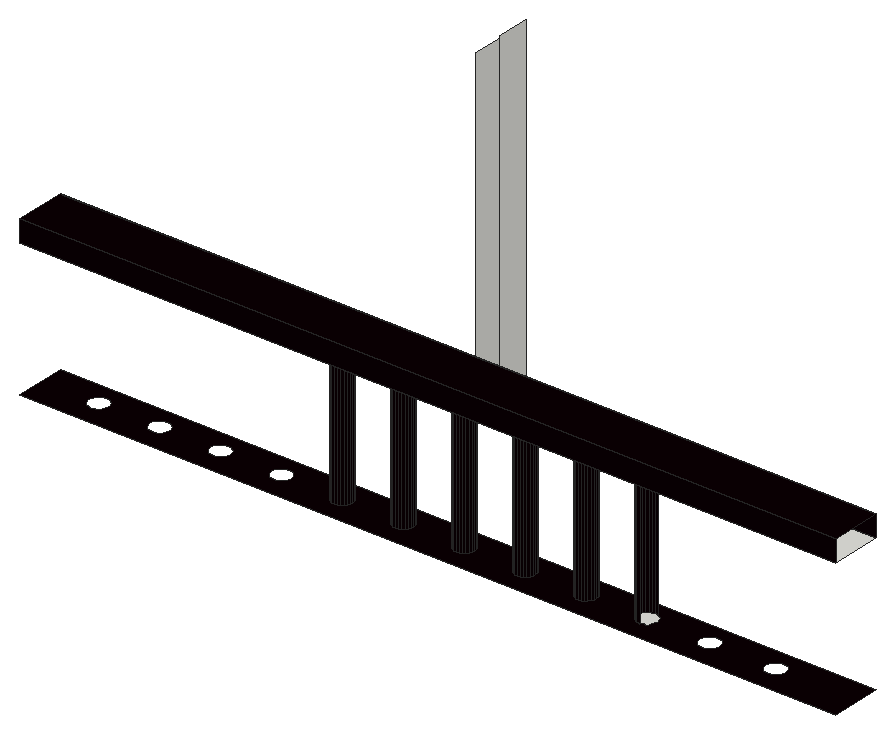
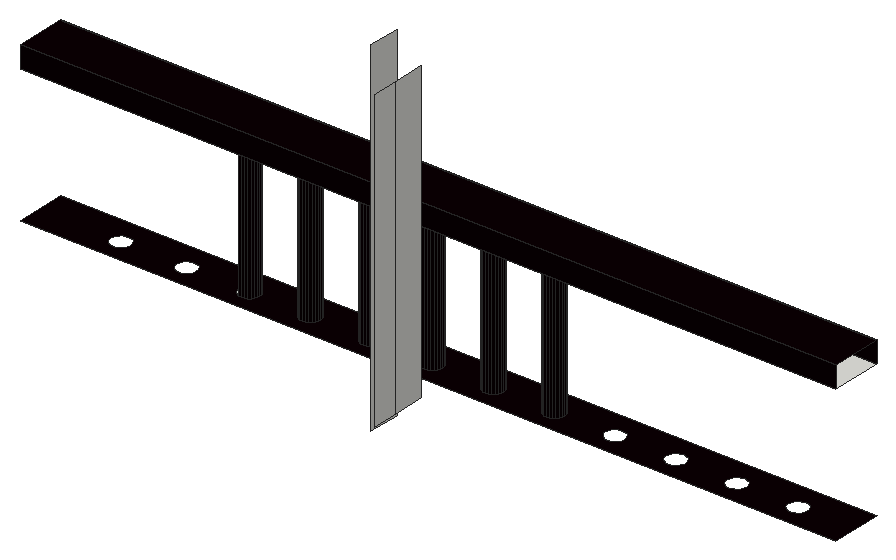
# SketchUp Ruby script. Lengths in inches.
U = 1.inch
M = Sketchup.active_model
def pt(a) = Geom::Point3d.new(a.map { |v| v * U })
def face(e, loops, mat)
  f = e.add_face(loops[0].map { |a| pt(a) })
  loops[1..].each { |l| e.add_face(l.map { |a| pt(a) }).erase! }
  f.material = f.back_material = mat if mat
  f
end
# faces: each face lists its corners as indices into pts; further lists are holes
def faces(e, pts, list, mat = nil) = list.each { |f| face(e, (f[0].is_a?(Array) ? f : [f]).map { |l| l.map { |i| pts[i] } }, mat) }
# xy, xz, yz: faces in a plane at the given z, y or x. An outline is a flat list of corners, or four numbers for a rectangle; further outlines are holes
def ring(l) = l.size == 4 ? [[l[0], l[1]], [l[2], l[1]], [l[2], l[3]], [l[0], l[3]]] : l.each_slice(2).to_a
def flat(e, list, mat, &to3) = list.each { |f| face(e, (f[0].is_a?(Array) ? f : [f]).map { |l| ring(l).map { |u, v| to3.(u, v) } }, mat) }
def xy(e, z, list, mat = nil) = flat(e, list, mat) { |x, y| [x, y, z] }
def xz(e, y, list, mat = nil) = flat(e, list, mat) { |x, z| [x, y, z] }
def yz(e, x, list, mat = nil) = flat(e, list, mat) { |y, z| [x, y, z] }
def lines(e, pts, list) = list.each { |a, b| e.add_line(pt(pts[a]), pt(pts[b])) }
# prism: a flat outline (further loops are holes) pulled along v
def prism(e, loops, v, mat = nil)
  f = face(e, loops, mat); d = Geom::Vector3d.new(v.map { |x| x * U })
  f.pushpull(f.normal.samedirection?(d) ? d.length : -d.length)
end
def box(e, o, s, mat = nil) = prism(e, [[o, [o[0] + s[0], o[1], o[2]], [o[0] + s[0], o[1] + s[1], o[2]], [o[0], o[1] + s[1], o[2]]]], [0, 0, s[2]], mat)
def at(x, y, z, deg = 0) = Geom::Transformation.translation(pt([x, y, z])) * Geom::Transformation.rotation(ORIGIN, Z_AXIS, deg.degrees)
def axes(o, x, y, z) = Geom::Transformation.new([*x, 0, *y, 0, *z, 0, *pt(o).to_a, 1])
def part(name) = M.definitions.add(name)
# library, detail: a bought-in or finely detailed component or shape, given as its bounding box
def library(name, o, s) = part(name).tap { |d| box(d.entities, o, s) }
def detail(e, o, s) = box(e.add_group.entities, o, s)
def put(e, d, t, mat = nil) = e.add_instance(d, t).tap { |i| i.material = mat if mat }
def group(e, t, mat = nil) = e.add_group.tap { |g| g.transformation = t; g.material = mat if mat }.entities
root = M.entities
M.materials.add("[Metal Seamed]").color = [11, 0, 4]
xy(root,300,[[437.97,74.99,437.36,75.05,436.8,75.25,436.3,75.6,435.91,76.06,435.66,76.61,435.55,77.2,435.6,77.8,435.81,78.37,436.16,78.86,436.62,79.25,437.16,79.51,437.76,79.61,438.36,79.5625,438.93,79.36,439.42,79.01,439.8125,78.55,440.07,78,440.17,77.41,440.12,76.81,439.91,76.24,439.57,75.74,439.11,75.36,438.56,75.1],[451.9,74.99,451.3,75.05,450.73,75.25,450.24,75.6,449.85,76.06,449.6,76.61,449.49,77.2,449.54,77.8,449.75,78.37,450.09,78.86,450.56,79.25,451.1,79.51,451.7,79.61,452.3,79.5625,452.87,79.36,453.36,79.01,453.75,78.55,454,78,454.11,77.41,454.06,76.81,453.85,76.24,453.51,75.74,453.04,75.36,452.5,75.1],[465.84,74.99,465.24,75.05,464.67,75.25,464.18,75.6,463.79,76.06,463.53,76.61,463.43,77.2,463.48,77.8,463.69,78.37,464.03,78.86,464.49,79.25,465.04,79.51,465.63,79.61,466.24,79.5625,466.8,79.36,467.3,79.01,467.6875,78.55,467.94,78,468.05,77.41,468,76.81,467.79,76.24,467.44,75.74,466.98,75.36,466.44,75.1],[479.78,74.99,479.18,75.05,478.61,75.25,478.11,75.6,477.73,76.06,477.47,76.61,477.36,77.2,477.42,77.8,477.62,78.37,477.97,78.86,478.43,79.25,478.98,79.51,479.57,79.61,480.17,79.5625,480.74,79.36,481.24,79.01,481.625,78.55,481.88,78,481.99,77.41,481.93,76.81,481.73,76.24,481.38,75.74,480.92,75.36,480.37,75.1],[493.72,74.99,493.11,75.05,492.55,75.25,492.05,75.6,491.66,76.06,491.41,76.61,491.3,77.2,491.35,77.8,491.56,78.37,491.91,78.86,492.37,79.25,492.91,79.51,493.51,79.61,494.11,79.5625,494.68,79.36,495.17,79.01,495.5625,78.55,495.82,78,495.92,77.41,495.87,76.81,495.66,76.24,495.32,75.74,494.86,75.36,494.31,75.1],
  [507.65,74.99,507.05,75.05,506.48,75.25,505.99,75.6,505.6,76.06,505.35,76.61,505.24,77.2,505.29,77.8,505.5,78.37,505.84,78.86,506.31,79.25,506.85,79.51,507.45,79.61,508.05,79.5625,508.62,79.36,509.11,79.01,509.5,78.55,509.75,78,509.86,77.41,509.81,76.81,509.6,76.24,509.26,75.74,508.79,75.36,508.25,75.1]])
xy(root,300,[[[369.3125,70.97,555.7,82.57],[382.22,74.99,381.61,75.05,381.05,75.25,380.55,75.6,380.16,76.06,379.91,76.61,379.8,77.2,379.85,77.8,380.06,78.37,380.41,78.86,380.87,79.25,381.41,79.51,382.01,79.61,382.61,79.5625,383.18,79.36,383.67,79.01,384.0625,78.55,384.32,78,384.42,77.41,384.37,76.81,384.16,76.24,383.82,75.74,383.36,75.36,382.81,75.1],[396.15,74.99,395.55,75.05,394.98,75.25,394.49,75.6,394.1,76.06,393.85,76.61,393.74,77.2,393.79,77.8,394,78.37,394.34,78.86,394.81,79.25,395.35,79.51,395.95,79.61,396.55,79.5625,397.12,79.36,397.61,79.01,398,78.55,398.25,78,398.36,77.41,398.31,76.81,398.1,76.24,397.76,75.74,397.29,75.36,396.75,75.1],[410.09,74.99,409.49,75.05,408.92,75.25,408.43,75.6,408.04,76.06,407.78,76.61,407.68,77.2,407.73,77.8,407.94,78.37,408.28,78.86,408.74,79.25,409.29,79.51,409.88,79.61,410.49,79.5625,411.05,79.36,411.55,79.01,411.9375,78.55,412.19,78,412.3,77.41,412.25,76.81,412.04,76.24,411.69,75.74,411.23,75.36,410.69,75.1],[424.03,74.99,423.43,75.05,422.86,75.25,422.36,75.6,421.98,76.06,421.72,76.61,421.61,77.2,421.67,77.8,421.87,78.37,422.22,78.86,422.68,79.25,423.23,79.51,423.82,79.61,424.42,79.5625,424.99,79.36,425.49,79.01,425.875,78.55,426.13,78,426.24,77.41,426.18,76.81,425.98,76.24,425.63,75.74,425.17,75.36,424.62,75.1],[437.97,74.99,437.36,75.05,436.8,75.25,436.3,75.6,435.91,76.06,435.66,76.61,435.55,77.2,435.6,77.8,435.81,78.37,436.16,78.86,436.62,79.25,437.16,79.51,437.76,79.61,438.36,79.5625,438.93,79.36,439.42,79.01,439.8125,78.55,440.07,78,440.17,77.41,440.12,76.81,439.91,76.24,439.57,75.74,439.11,75.36,438.56,75.1],[451.9,74.99,451.3,75.05,450.73,75.25,450.24,75.6,449.85,76.06,449.6,76.61,449.49,77.2,449.54,77.8,449.75,78.37,450.09,78.86,450.56,79.25,451.1,79.51,451.7,79.61,452.3,79.5625,452.87,79.36,453.36,79.01,453.75,78.55,454,78,454.11,77.41,454.06,76.81,453.85,76.24,453.51,75.74,453.04,75.36,452.5,75.1],[465.84,74.99,465.24,75.05,464.67,75.25,464.18,75.6,463.79,76.06,463.53,76.61,463.43,77.2,463.48,77.8,463.69,78.37,464.03,78.86,464.49,79.25,465.04,79.51,465.63,79.61,466.24,79.5625,466.8,79.36,467.3,79.01,467.6875,78.55,467.94,78,468.05,77.41,468,76.81,467.79,76.24,467.44,75.74,466.98,75.36,466.44,75.1],[479.78,74.99,479.18,75.05,478.61,75.25,478.11,75.6,477.73,76.06,477.47,76.61,477.36,77.2,477.42,77.8,477.62,78.37,477.97,78.86,478.43,79.25,478.98,79.51,479.57,79.61,480.17,79.5625,480.74,79.36,481.24,79.01,481.625,78.55,481.88,78,481.99,77.41,481.93,76.81,481.73,76.24,481.38,75.74,480.92,75.36,480.37,75.1],[493.72,74.99,493.11,75.05,492.55,75.25,492.05,75.6,491.66,76.06,491.41,76.61,491.3,77.2,491.35,77.8,491.56,78.37,491.91,78.86,492.37,79.25,492.91,79.51,493.51,79.61,494.11,79.5625,494.68,79.36,495.17,79.01,495.5625,78.55,495.82,78,495.92,77.41,495.87,76.81,495.66,76.24,495.32,75.74,494.86,75.36,494.31,75.1],[507.65,74.99,507.05,75.05,506.48,75.25,505.99,75.6,505.6,76.06,505.35,76.61,505.24,77.2,505.29,77.8,505.5,78.37,505.84,78.86,506.31,79.25,506.85,79.51,507.45,79.61,508.05,79.5625,508.62,79.36,509.11,79.01,509.5,78.55,509.75,78,509.86,77.41,509.81,76.81,509.6,76.24,509.26,75.74,508.79,75.36,508.25,75.1],[521.97,74.99,521.36,75.05,520.8,75.25,520.3,75.6,519.91,76.06,519.66,76.61,519.55,77.2,519.6,77.8,519.81,78.37,520.16,78.86,520.62,79.25,521.16,79.51,521.76,79.61,522.36,79.5625,522.93,79.36,523.42,79.01,523.8125,78.55,524.07,78,524.17,77.41,524.12,76.81,523.91,76.24,523.57,75.74,523.11,75.36,522.56,75.1],[537.09,74.99,536.49,75.05,535.92,75.25,535.43,75.6,535.04,76.06,534.78,76.61,534.68,77.2,534.73,77.8,534.94,78.37,535.28,78.86,535.74,79.25,536.29,79.51,536.88,79.61,537.49,79.5625,538.05,79.36,538.55,79.01,538.9375,78.55,539.19,78,539.3,77.41,539.25,76.81,539.04,76.24,538.69,75.74,538.23,75.36,537.69,75.1]]],"[Metal Seamed]")
xy(root,331.08,[[[369.3125,70.97,555.7,82.57],[382.22,74.99,382.81,75.1,383.36,75.36,383.82,75.74,384.16,76.24,384.37,76.81,384.42,77.41,384.32,78,384.0625,78.55,383.67,79.01,383.18,79.36,382.61,79.5625,382.01,79.61,381.41,79.51,380.87,79.25,380.41,78.86,380.06,78.37,379.85,77.8,379.8,77.2,379.91,76.61,380.16,76.06,380.55,75.6,381.05,75.25,381.61,75.05],[424.03,74.99,424.62,75.1,425.17,75.36,425.63,75.74,425.98,76.24,426.18,76.81,426.24,77.41,426.13,78,425.875,78.55,425.49,79.01,424.99,79.36,424.42,79.5625,423.82,79.61,423.23,79.51,422.68,79.25,422.22,78.86,421.87,78.37,421.67,77.8,421.61,77.2,421.72,76.61,421.98,76.06,422.36,75.6,422.86,75.25,423.43,75.05]]])
xy(root,331.3125,[[451.9,74.99,452.5,75.1,453.04,75.36,453.51,75.74,453.85,76.24,454.06,76.81,454.11,77.41,454,78,453.75,78.55,453.36,79.01,452.87,79.36,452.3,79.5625,451.7,79.61,451.1,79.51,450.56,79.25,450.09,78.86,449.75,78.37,449.54,77.8,449.49,77.2,449.6,76.61,449.85,76.06,450.24,75.6,450.73,75.25,451.3,75.05]])
xy(root,331.6875,[[465.84,74.99,466.44,75.1,466.98,75.36,467.44,75.74,467.79,76.24,468,76.81,468.05,77.41,467.94,78,467.6875,78.55,467.3,79.01,466.8,79.36,466.24,79.5625,465.63,79.61,465.04,79.51,464.49,79.25,464.03,78.86,463.69,78.37,463.48,77.8,463.43,77.2,463.53,76.61,463.79,76.06,464.18,75.6,464.67,75.25,465.24,75.05]])
xy(root,331.75,[[437.97,74.99,438.56,75.1,439.11,75.36,439.57,75.74,439.91,76.24,440.12,76.81,440.17,77.41,440.07,78,439.8125,78.55,439.42,79.01,438.93,79.36,438.36,79.5625,437.76,79.61,437.16,79.51,436.62,79.25,436.16,78.86,435.81,78.37,435.6,77.8,435.55,77.2,435.66,76.61,435.91,76.06,436.3,75.6,436.8,75.25,437.36,75.05]])
xy(root,332.0625,[[493.72,74.99,494.31,75.1,494.86,75.36,495.32,75.74,495.66,76.24,495.87,76.81,495.92,77.41,495.82,78,495.5625,78.55,495.17,79.01,494.68,79.36,494.11,79.5625,493.51,79.61,492.91,79.51,492.37,79.25,491.91,78.86,491.56,78.37,491.35,77.8,491.3,77.2,491.41,76.61,491.66,76.06,492.05,75.6,492.55,75.25,493.11,75.05]])
xy(root,332.1875,[[479.78,74.99,480.37,75.1,480.92,75.36,481.38,75.74,481.73,76.24,481.93,76.81,481.99,77.41,481.88,78,481.625,78.55,481.24,79.01,480.74,79.36,480.17,79.5625,479.57,79.61,478.98,79.51,478.43,79.25,477.97,78.86,477.62,78.37,477.42,77.8,477.36,77.2,477.47,76.61,477.73,76.06,478.11,75.6,478.61,75.25,479.18,75.05]])
xy(root,332.875,[[507.65,74.99,508.25,75.1,508.79,75.36,509.26,75.74,509.6,76.24,509.81,76.81,509.86,77.41,509.75,78,509.5,78.55,509.11,79.01,508.62,79.36,508.05,79.5625,507.45,79.61,506.85,79.51,506.31,79.25,505.84,78.86,505.5,78.37,505.29,77.8,505.24,77.2,505.35,76.61,505.6,76.06,505.99,75.6,506.48,75.25,507.05,75.05]])
xy(root,336,[[369.3125,70.97,555.7,82.57]],"[Metal Seamed]")
xz(root,70.97,[[369.3125,331.08,555.7,336]],"[Metal Seamed]")
xz(root,82.57,[[369.3125,331.08,555.7,336]],"[Metal Seamed]")
yz(root,445.08,[[106.41,313.04,113.66,380.98],[113.66,313.04,119.66,380.98]])
yz(root,450.64,[[106.41,307.48,113.66,386.54]])
p = [[436.8,75.25,300],[437.36,75.05,300],[437.36,75.05,331.75],[436.8,75.25,331.75],[437.97,74.99,300],[437.97,74.99,331.75],
  [438.56,75.1,300],[438.56,75.1,331.75],[450.73,75.25,300],[451.3,75.05,300],[451.3,75.05,331.3125],[450.73,75.25,331.3125],
  [451.9,74.99,300],[451.9,74.99,331.3125],[452.5,75.1,300],[452.5,75.1,331.3125],[464.67,75.25,300],[465.24,75.05,300],
  [465.24,75.05,331.6875],[464.67,75.25,331.6875],[465.84,74.99,300],[465.84,74.99,331.6875],[466.44,75.1,300],[466.44,75.1,331.6875],
  [478.61,75.25,300],[479.18,75.05,300],[479.18,75.05,332.1875],[478.61,75.25,332.1875],[479.78,74.99,300],[479.78,74.99,332.1875],
  [480.37,75.1,300],[480.37,75.1,332.1875],[492.55,75.25,300],[493.11,75.05,300],[493.11,75.05,332.0625],[492.55,75.25,332.0625],
  [493.72,74.99,300],[493.72,74.99,332.0625],[494.31,75.1,300],[494.31,75.1,332.0625],[506.48,75.25,300],[507.05,75.05,300],
  [507.05,75.05,332.875],[506.48,75.25,332.875],[507.65,74.99,300],[507.65,74.99,332.875],[439.11,75.36,300],[439.11,75.36,331.75],
  [453.04,75.36,300],[453.04,75.36,331.3125],[466.98,75.36,300],[466.98,75.36,331.6875],[480.92,75.36,300],[480.92,75.36,332.1875],
  [494.86,75.36,300],[494.86,75.36,332.0625],[436.3,75.6,300],[436.3,75.6,331.75],[450.24,75.6,300],[450.24,75.6,331.3125],
  [464.18,75.6,300],[464.18,75.6,331.6875],[478.11,75.6,300],[478.11,75.6,332.1875],[492.05,75.6,300],[492.05,75.6,332.0625],
  [505.99,75.6,300],[505.99,75.6,332.875],[439.57,75.74,300],[439.57,75.74,331.75],[453.51,75.74,300],[453.51,75.74,331.3125],
  [467.44,75.74,300],[467.44,75.74,331.6875],[481.38,75.74,300],[481.38,75.74,332.1875],[495.32,75.74,300],[495.32,75.74,332.0625],
  [435.91,76.06,300],[435.91,76.06,331.75],[449.85,76.06,300],[449.85,76.06,331.3125],[463.79,76.06,300],[463.79,76.06,331.6875],
  [477.73,76.06,300],[477.73,76.06,332.1875],[491.66,76.06,300],[491.66,76.06,332.0625],[505.6,76.06,300],[505.6,76.06,332.875],
  [439.91,76.24,300],[439.91,76.24,331.75],[453.85,76.24,300],[453.85,76.24,331.3125],[467.79,76.24,300],[467.79,76.24,331.6875],
  [481.73,76.24,300],[481.73,76.24,332.1875],[495.66,76.24,300],[495.66,76.24,332.0625],[435.66,76.61,300],[435.66,76.61,331.75],
  [449.6,76.61,300],[449.6,76.61,331.3125],[463.53,76.61,300],[463.53,76.61,331.6875],[477.47,76.61,300],[477.47,76.61,332.1875],
  [491.41,76.61,300],[491.41,76.61,332.0625],[505.35,76.61,300],[505.35,76.61,332.875],[440.12,76.81,300],[440.12,76.81,331.75],
  [454.06,76.81,300],[454.06,76.81,331.3125],[468,76.81,300],[468,76.81,331.6875],[481.93,76.81,300],[481.93,76.81,332.1875],
  [495.87,76.81,300],[495.87,76.81,332.0625],[435.55,77.2,300],[435.55,77.2,331.75],[449.49,77.2,300],[449.49,77.2,331.3125],
  [463.43,77.2,300],[463.43,77.2,331.6875],[477.36,77.2,300],[477.36,77.2,332.1875],[491.3,77.2,300],[491.3,77.2,332.0625],
  [505.24,77.2,300],[505.24,77.2,332.875],[440.17,77.41,300],[440.17,77.41,331.75],[454.11,77.41,300],[454.11,77.41,331.3125],
  [468.05,77.41,300],[468.05,77.41,331.6875],[481.99,77.41,300],[481.99,77.41,332.1875],[495.92,77.41,300],[495.92,77.41,332.0625],
  [435.6,77.8,300],[435.6,77.8,331.75],[449.54,77.8,300],[449.54,77.8,331.3125],[463.48,77.8,300],[463.48,77.8,331.6875],
  [477.42,77.8,300],[477.42,77.8,332.1875],[491.35,77.8,300],[491.35,77.8,332.0625],[505.29,77.8,300],[505.29,77.8,332.875],
  [440.07,78,300],[440.07,78,331.75],[454,78,300],[454,78,331.3125],[467.94,78,300],[467.94,78,331.6875],
  [481.88,78,300],[481.88,78,332.1875],[495.82,78,300],[495.82,78,332.0625],[435.81,78.37,300],[435.81,78.37,331.75],
  [449.75,78.37,300],[449.75,78.37,331.3125],[463.69,78.37,300],[463.69,78.37,331.6875],[477.62,78.37,300],[477.62,78.37,332.1875],
  [491.56,78.37,300],[491.56,78.37,332.0625],[505.5,78.37,300],[505.5,78.37,332.875],[439.8125,78.55,300],[439.8125,78.55,331.75],
  [453.75,78.55,300],[453.75,78.55,331.3125],[467.6875,78.55,300],[467.6875,78.55,331.6875],[481.625,78.55,300],[481.625,78.55,332.1875],
  [495.5625,78.55,300],[495.5625,78.55,332.0625],[436.16,78.86,300],[436.16,78.86,331.75],[450.09,78.86,300],[450.09,78.86,331.3125],
  [464.03,78.86,300],[464.03,78.86,331.6875],[477.97,78.86,300],[477.97,78.86,332.1875],[491.91,78.86,300],[491.91,78.86,332.0625],
  [505.84,78.86,300],[505.84,78.86,332.875],[439.42,79.01,300],[439.42,79.01,331.75],[453.36,79.01,300],[453.36,79.01,331.3125],
  [467.3,79.01,300],[467.3,79.01,331.6875],[481.24,79.01,300],[481.24,79.01,332.1875],[495.17,79.01,300],[495.17,79.01,332.0625],
  [436.62,79.25,300],[436.62,79.25,331.75],[450.56,79.25,300],[450.56,79.25,331.3125],[464.49,79.25,300],[464.49,79.25,331.6875],
  [478.43,79.25,300],[478.43,79.25,332.1875],[492.37,79.25,300],[492.37,79.25,332.0625],[506.31,79.25,300],[506.31,79.25,332.875],
  [438.93,79.36,300],[438.93,79.36,331.75],[452.87,79.36,300],[452.87,79.36,331.3125],[466.8,79.36,300],[466.8,79.36,331.6875],
  [480.74,79.36,300],[480.74,79.36,332.1875],[494.68,79.36,300],[494.68,79.36,332.0625],[437.16,79.51,300],[437.16,79.51,331.75],
  [451.1,79.51,300],[451.1,79.51,331.3125],[465.04,79.51,300],[465.04,79.51,331.6875],[478.98,79.51,300],[478.98,79.51,332.1875],
  [492.91,79.51,300],[492.91,79.51,332.0625],[506.85,79.51,300],[506.85,79.51,332.875],[438.36,79.5625,300],[438.36,79.5625,331.75],
  [452.3,79.5625,300],[452.3,79.5625,331.3125],[466.24,79.5625,300],[466.24,79.5625,331.6875],[480.17,79.5625,300],[480.17,79.5625,332.1875],
  [494.11,79.5625,300],[494.11,79.5625,332.0625],[437.76,79.61,300],[437.76,79.61,331.75],[451.7,79.61,300],[451.7,79.61,331.3125],
  [465.63,79.61,300],[465.63,79.61,331.6875],[479.57,79.61,300],[479.57,79.61,332.1875],[493.51,79.61,300],[493.51,79.61,332.0625],
  [507.45,79.61,300],[507.45,79.61,332.875],[508.05,79.5625,300],[508.05,79.5625,332.875]]
faces(root,p,[[0,1,2,3],[1,4,5,2],[4,6,7,5],[8,9,10,11],[9,12,13,10],[12,14,15,13],[16,17,18,19],[17,20,21,18],
  [20,22,23,21],[24,25,26,27],[25,28,29,26],[28,30,31,29],[32,33,34,35],[33,36,37,34],[36,38,39,37],[40,41,42,43],
  [41,44,45,42],[6,46,47,7],[14,48,49,15],[22,50,51,23],[30,52,53,31],[38,54,55,39],[56,0,3,57],[58,8,11,59],
  [60,16,19,61],[62,24,27,63],[64,32,35,65],[66,40,43,67],[46,68,69,47],[48,70,71,49],[50,72,73,51],[52,74,75,53],
  [54,76,77,55],[78,56,57,79],[80,58,59,81],[82,60,61,83],[84,62,63,85],[86,64,65,87],[88,66,67,89],[68,90,91,69],
  [70,92,93,71],[72,94,95,73],[74,96,97,75],[76,98,99,77],[100,78,79,101],[102,80,81,103],[104,82,83,105],[106,84,85,107],
  [108,86,87,109],[110,88,89,111],[90,112,113,91],[92,114,115,93],[94,116,117,95],[96,118,119,97],[98,120,121,99],[122,100,101,123],
  [124,102,103,125],[126,104,105,127],[128,106,107,129],[130,108,109,131],[132,110,111,133],[112,134,135,113],[114,136,137,115],[116,138,139,117],
  [118,140,141,119],[120,142,143,121],[144,122,123,145],[146,124,125,147],[148,126,127,149],[150,128,129,151],[152,130,131,153],[154,132,133,155],
  [134,156,157,135],[136,158,159,137],[138,160,161,139],[140,162,163,141],[142,164,165,143],[166,144,145,167],[168,146,147,169],[170,148,149,171],
  [172,150,151,173],[174,152,153,175],[176,154,155,177],[156,178,179,157],[158,180,181,159],[160,182,183,161],[162,184,185,163],[164,186,187,165],
  [188,166,167,189],[190,168,169,191],[192,170,171,193],[194,172,173,195],[196,174,175,197],[198,176,177,199],[178,200,201,179],[180,202,203,181],
  [182,204,205,183],[184,206,207,185],[186,208,209,187],[210,188,189,211],[212,190,191,213],[214,192,193,215],[216,194,195,217],[218,196,197,219],
  [220,198,199,221],[200,222,223,201],[202,224,225,203],[204,226,227,205],[206,228,229,207],[208,230,231,209],[232,210,211,233],[234,212,213,235],
  [236,214,215,237],[238,216,217,239],[240,218,219,241],[242,220,221,243],[222,244,245,223],[224,246,247,225],[226,248,249,227],[228,250,251,229],
  [230,252,253,231],[254,232,233,255],[256,234,235,257],[258,236,237,259],[260,238,239,261],[262,240,241,263],[264,242,243,265],[244,254,255,245],
  [246,256,257,247],[248,258,259,249],[250,260,261,251],[252,262,263,253],[266,264,265,267]],"[Metal Seamed]")
